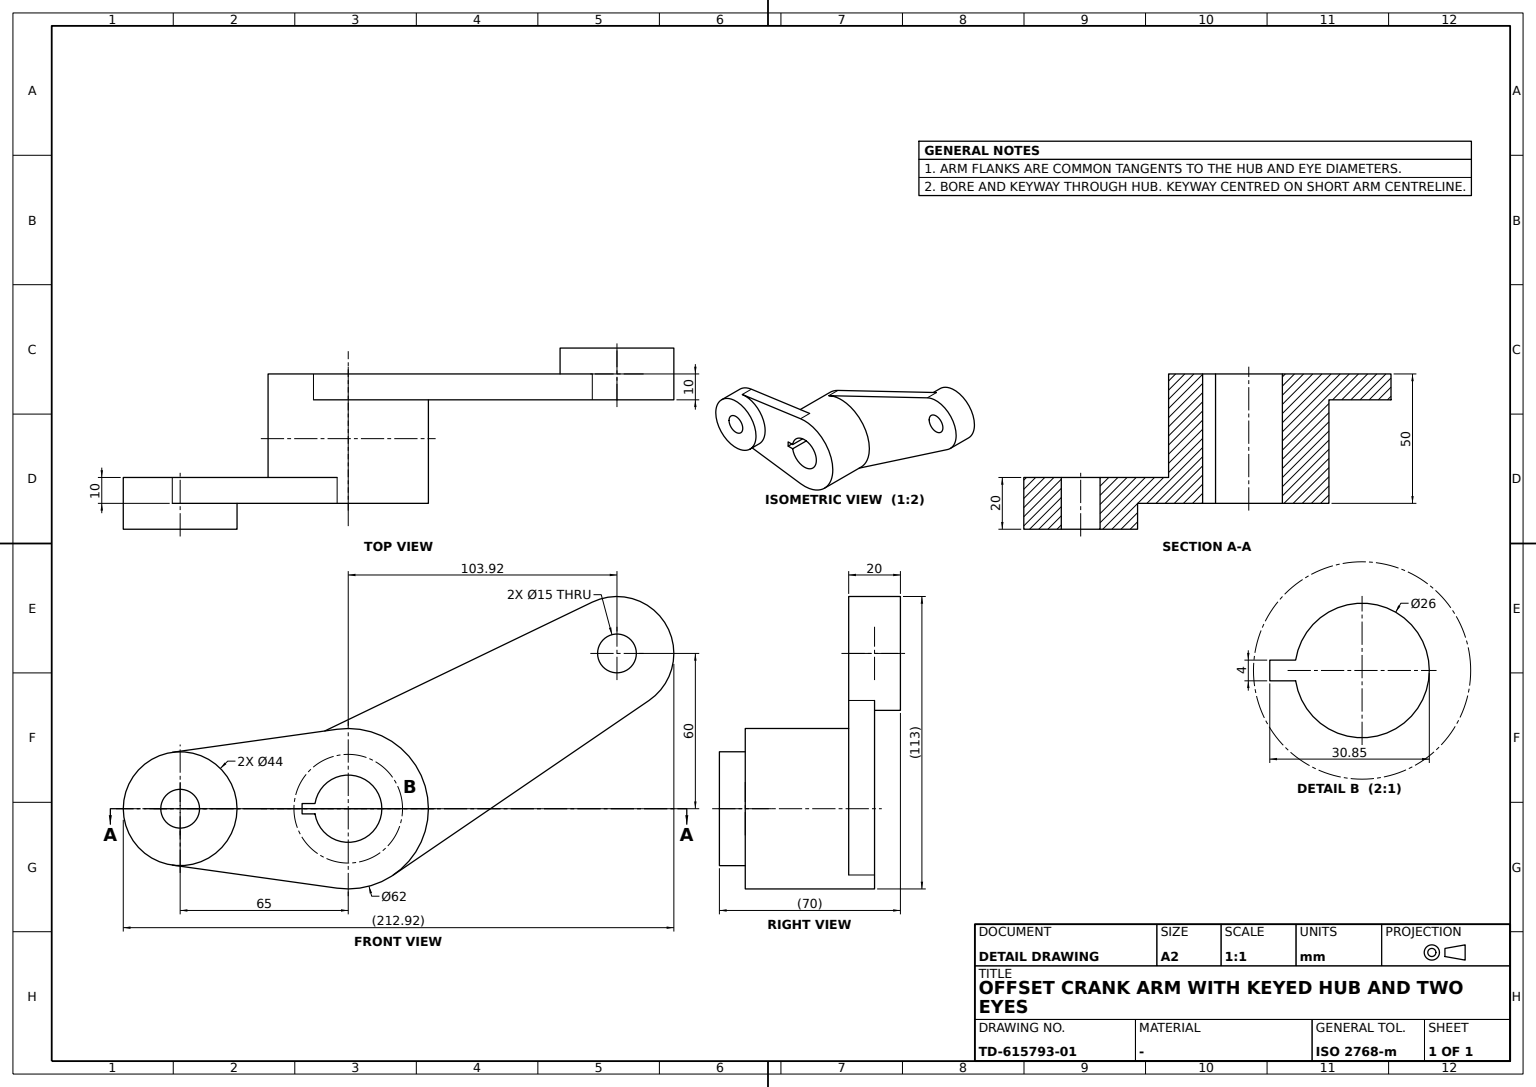
ISO-10303-21;
HEADER;
FILE_DESCRIPTION((''),'2;1');
FILE_NAME('','',(''),(''),'','','');
FILE_SCHEMA(('AUTOMOTIVE_DESIGN'));
ENDSEC;
DATA;
#1=APPLICATION_CONTEXT('');
#2=PRODUCT_CONTEXT('',#1,'mechanical');
#3=PRODUCT('','','',(#2));
#4=PRODUCT_DEFINITION_FORMATION('','',#3);
#5=PRODUCT_DEFINITION_CONTEXT('',#1,'design');
#6=PRODUCT_DEFINITION('','',#4,#5);
#7=PRODUCT_DEFINITION_SHAPE('','',#6);
#8=(LENGTH_UNIT()NAMED_UNIT(*)SI_UNIT(.MILLI.,.METRE.));
#9=(NAMED_UNIT(*)PLANE_ANGLE_UNIT()SI_UNIT($,.RADIAN.));
#10=(NAMED_UNIT(*)SI_UNIT($,.STERADIAN.)SOLID_ANGLE_UNIT());
#11=UNCERTAINTY_MEASURE_WITH_UNIT(LENGTH_MEASURE(0.005),#8,'distance_accuracy_value','');
#12=(GEOMETRIC_REPRESENTATION_CONTEXT(3)GLOBAL_UNCERTAINTY_ASSIGNED_CONTEXT((#11))GLOBAL_UNIT_ASSIGNED_CONTEXT((#8,#9,#10))REPRESENTATION_CONTEXT('',''));
#13=CARTESIAN_POINT('',(-17.469854,25.608674,10.));
#14=VERTEX_POINT('',#13);
#15=CARTESIAN_POINT('',(-17.469854,25.608674,0.));
#16=VERTEX_POINT('',#15);
#17=DIRECTION('',(0.,0.,-1.));
#18=VECTOR('',#17,1000.);
#19=LINE('',#13,#18);
#20=EDGE_CURVE('',#14,#16,#19,.T.);
#21=ORIENTED_EDGE('',*,*,#20,.T.);
#22=CARTESIAN_POINT('',(-116.321009,-41.826102,0.));
#23=VERTEX_POINT('',#22);
#24=DIRECTION('',(-0.826086272,-0.563543672,0.));
#25=VECTOR('',#24,1000.);
#26=LINE('',#15,#25);
#27=EDGE_CURVE('',#16,#23,#26,.T.);
#28=ORIENTED_EDGE('',*,*,#27,.T.);
#29=CARTESIAN_POINT('',(-116.321009,-41.826102,10.));
#30=VERTEX_POINT('',#29);
#31=LINE('',#29,#18);
#32=EDGE_CURVE('',#30,#23,#31,.T.);
#33=ORIENTED_EDGE('',*,*,#32,.F.);
#34=LINE('',#13,#25);
#35=EDGE_CURVE('',#14,#30,#34,.T.);
#36=ORIENTED_EDGE('',*,*,#35,.F.);
#37=EDGE_LOOP('',(#21,#28,#33,#36));
#38=FACE_BOUND('',#37,.T.);
#39=DIRECTION('',(0.563543672,-0.826086272,0.));
#40=DIRECTION('',(0.826086272,0.563543672,0.));
#41=AXIS2_PLACEMENT_3D('',#13,#39,#40);
#42=PLANE('',#41);
#43=ADVANCED_FACE('',(#38),#42,.F.);
#44=CARTESIAN_POINT('',(43.,0.,60.));
#45=VERTEX_POINT('',#44);
#46=CARTESIAN_POINT('',(87.,0.,60.));
#47=VERTEX_POINT('',#46);
#48=CARTESIAN_POINT('',(65.,0.,60.));
#49=DIRECTION('',(0.,0.,1.));
#50=DIRECTION('',(1.,0.,0.));
#51=AXIS2_PLACEMENT_3D('',#48,#49,#50);
#52=CIRCLE('',#51,22.);
#53=EDGE_CURVE('',#45,#47,#52,.T.);
#54=ORIENTED_EDGE('',*,*,#53,.F.);
#55=CARTESIAN_POINT('',(43.,0.,50.));
#56=VERTEX_POINT('',#55);
#57=CARTESIAN_POINT('',(43.,0.,40.));
#58=VECTOR('',#49,1000.);
#59=LINE('',#57,#58);
#60=EDGE_CURVE('',#45,#56,#59,.F.);
#61=ORIENTED_EDGE('',*,*,#60,.T.);
#62=CARTESIAN_POINT('',(68.046154,-21.788092,50.));
#63=VERTEX_POINT('',#62);
#64=CARTESIAN_POINT('',(65.,0.,50.));
#65=AXIS2_PLACEMENT_3D('',#64,#17,#50);
#66=CIRCLE('',#65,22.);
#67=EDGE_CURVE('',#63,#56,#66,.T.);
#68=ORIENTED_EDGE('',*,*,#67,.F.);
#69=CARTESIAN_POINT('',(68.046154,-21.788092,40.));
#70=VERTEX_POINT('',#69);
#71=LINE('',#69,#58);
#72=EDGE_CURVE('',#70,#63,#71,.T.);
#73=ORIENTED_EDGE('',*,*,#72,.F.);
#74=CARTESIAN_POINT('',(87.,0.,40.));
#75=VERTEX_POINT('',#74);
#76=CARTESIAN_POINT('',(65.,0.,40.));
#77=AXIS2_PLACEMENT_3D('',#76,#49,#50);
#78=CIRCLE('',#77,22.);
#79=EDGE_CURVE('',#70,#75,#78,.T.);
#80=ORIENTED_EDGE('',*,*,#79,.T.);
#81=LINE('',#74,#58);
#82=EDGE_CURVE('',#75,#47,#81,.T.);
#83=ORIENTED_EDGE('',*,*,#82,.T.);
#84=EDGE_LOOP('',(#54,#61,#68,#73,#80,#83));
#85=FACE_BOUND('',#84,.T.);
#86=CYLINDRICAL_SURFACE('',#77,22.);
#87=ADVANCED_FACE('',(#85),#86,.T.);
#88=CARTESIAN_POINT('',(68.046154,21.788092,40.));
#89=VERTEX_POINT('',#88);
#90=CARTESIAN_POINT('',(68.046154,21.788092,50.));
#91=VERTEX_POINT('',#90);
#92=LINE('',#88,#58);
#93=EDGE_CURVE('',#89,#91,#92,.T.);
#94=ORIENTED_EDGE('',*,*,#93,.T.);
#95=EDGE_CURVE('',#56,#91,#66,.T.);
#96=ORIENTED_EDGE('',*,*,#95,.F.);
#97=ORIENTED_EDGE('',*,*,#60,.F.);
#98=EDGE_CURVE('',#47,#45,#52,.T.);
#99=ORIENTED_EDGE('',*,*,#98,.F.);
#100=ORIENTED_EDGE('',*,*,#82,.F.);
#101=EDGE_CURVE('',#75,#89,#78,.T.);
#102=ORIENTED_EDGE('',*,*,#101,.T.);
#103=EDGE_LOOP('',(#94,#96,#97,#99,#100,#102));
#104=FACE_BOUND('',#103,.T.);
#105=ADVANCED_FACE('',(#104),#86,.T.);
#106=CARTESIAN_POINT('',(-94.382971,-79.823898,0.));
#107=VERTEX_POINT('',#106);
#108=CARTESIAN_POINT('',(13.442836,-27.933674,0.));
#109=VERTEX_POINT('',#108);
#110=DIRECTION('',(0.901086272,0.433639862,0.));
#111=VECTOR('',#110,1000.);
#112=LINE('',#106,#111);
#113=EDGE_CURVE('',#107,#109,#112,.T.);
#114=ORIENTED_EDGE('',*,*,#113,.F.);
#115=CARTESIAN_POINT('',(-81.923048,-60.,0.));
#116=VERTEX_POINT('',#115);
#117=CARTESIAN_POINT('',(-103.923048,-60.,0.));
#118=AXIS2_PLACEMENT_3D('',#117,#17,#50);
#119=CIRCLE('',#118,22.);
#120=EDGE_CURVE('',#116,#107,#119,.T.);
#121=ORIENTED_EDGE('',*,*,#120,.F.);
#122=EDGE_CURVE('',#23,#116,#119,.T.);
#123=ORIENTED_EDGE('',*,*,#122,.F.);
#124=ORIENTED_EDGE('',*,*,#27,.F.);
#125=CARTESIAN_POINT('',(31.,0.,0.));
#126=VERTEX_POINT('',#125);
#127=CARTESIAN_POINT('',(0.,0.,0.));
#128=AXIS2_PLACEMENT_3D('',#127,#49,#50);
#129=CIRCLE('',#128,31.);
#130=EDGE_CURVE('',#126,#16,#129,.T.);
#131=ORIENTED_EDGE('',*,*,#130,.F.);
#132=EDGE_CURVE('',#109,#126,#129,.T.);
#133=ORIENTED_EDGE('',*,*,#132,.F.);
#134=EDGE_LOOP('',(#114,#121,#123,#124,#131,#133));
#135=FACE_BOUND('',#134,.T.);
#136=CARTESIAN_POINT('',(17.845233,2.,0.));
#137=VERTEX_POINT('',#136);
#138=CARTESIAN_POINT('',(12.845233,2.,0.));
#139=VERTEX_POINT('',#138);
#140=DIRECTION('',(-1.,0.,0.));
#141=VECTOR('',#140,1000.);
#142=LINE('',#136,#141);
#143=EDGE_CURVE('',#137,#139,#142,.T.);
#144=ORIENTED_EDGE('',*,*,#143,.T.);
#145=CARTESIAN_POINT('',(12.845233,-2.,0.));
#146=VERTEX_POINT('',#145);
#147=CIRCLE('',#128,13.);
#148=EDGE_CURVE('',#139,#146,#147,.T.);
#149=ORIENTED_EDGE('',*,*,#148,.T.);
#150=CARTESIAN_POINT('',(17.845233,-2.,0.));
#151=VERTEX_POINT('',#150);
#152=VECTOR('',#50,1000.);
#153=LINE('',#145,#152);
#154=EDGE_CURVE('',#146,#151,#153,.T.);
#155=ORIENTED_EDGE('',*,*,#154,.T.);
#156=DIRECTION('',(0.,1.,0.));
#157=VECTOR('',#156,1000.);
#158=LINE('',#150,#157);
#159=EDGE_CURVE('',#151,#137,#158,.T.);
#160=ORIENTED_EDGE('',*,*,#159,.T.);
#161=EDGE_LOOP('',(#144,#149,#155,#160));
#162=FACE_BOUND('',#161,.T.);
#163=PLANE('',#128);
#164=ADVANCED_FACE('',(#135,#162),#163,.F.);
#165=CARTESIAN_POINT('',(-96.423048,-60.,10.));
#166=VERTEX_POINT('',#165);
#167=CARTESIAN_POINT('',(-111.423048,-60.,10.));
#168=VERTEX_POINT('',#167);
#169=CARTESIAN_POINT('',(-103.923048,-60.,10.));
#170=AXIS2_PLACEMENT_3D('',#169,#17,#140);
#171=CIRCLE('',#170,7.5);
#172=EDGE_CURVE('',#166,#168,#171,.T.);
#173=ORIENTED_EDGE('',*,*,#172,.F.);
#174=CARTESIAN_POINT('',(-96.423048,-60.,-10.));
#175=VERTEX_POINT('',#174);
#176=LINE('',#165,#18);
#177=EDGE_CURVE('',#166,#175,#176,.T.);
#178=ORIENTED_EDGE('',*,*,#177,.T.);
#179=CARTESIAN_POINT('',(-111.423048,-60.,-10.));
#180=VERTEX_POINT('',#179);
#181=CARTESIAN_POINT('',(-103.923048,-60.,-10.));
#182=AXIS2_PLACEMENT_3D('',#181,#17,#140);
#183=CIRCLE('',#182,7.5);
#184=EDGE_CURVE('',#175,#180,#183,.T.);
#185=ORIENTED_EDGE('',*,*,#184,.T.);
#186=LINE('',#167,#18);
#187=EDGE_CURVE('',#180,#168,#186,.F.);
#188=ORIENTED_EDGE('',*,*,#187,.T.);
#189=EDGE_LOOP('',(#173,#178,#185,#188));
#190=FACE_BOUND('',#189,.T.);
#191=CYLINDRICAL_SURFACE('',#170,7.5);
#192=ADVANCED_FACE('',(#190),#191,.F.);
#193=CARTESIAN_POINT('',(-94.382971,-79.823898,10.));
#194=VERTEX_POINT('',#193);
#195=LINE('',#193,#18);
#196=EDGE_CURVE('',#194,#107,#195,.T.);
#197=ORIENTED_EDGE('',*,*,#196,.F.);
#198=CARTESIAN_POINT('',(-125.923048,-60.,10.));
#199=VERTEX_POINT('',#198);
#200=AXIS2_PLACEMENT_3D('',#169,#49,#50);
#201=CIRCLE('',#200,22.);
#202=EDGE_CURVE('',#199,#194,#201,.T.);
#203=ORIENTED_EDGE('',*,*,#202,.F.);
#204=CARTESIAN_POINT('',(-125.923048,-60.,-10.));
#205=VERTEX_POINT('',#204);
#206=LINE('',#198,#18);
#207=EDGE_CURVE('',#205,#199,#206,.F.);
#208=ORIENTED_EDGE('',*,*,#207,.F.);
#209=CARTESIAN_POINT('',(-81.923048,-60.,-10.));
#210=VERTEX_POINT('',#209);
#211=AXIS2_PLACEMENT_3D('',#181,#49,#50);
#212=CIRCLE('',#211,22.);
#213=EDGE_CURVE('',#205,#210,#212,.T.);
#214=ORIENTED_EDGE('',*,*,#213,.T.);
#215=CARTESIAN_POINT('',(-81.923048,-60.,10.));
#216=LINE('',#215,#18);
#217=EDGE_CURVE('',#116,#210,#216,.T.);
#218=ORIENTED_EDGE('',*,*,#217,.F.);
#219=ORIENTED_EDGE('',*,*,#120,.T.);
#220=EDGE_LOOP('',(#197,#203,#208,#214,#218,#219));
#221=FACE_BOUND('',#220,.T.);
#222=CYLINDRICAL_SURFACE('',#170,22.);
#223=ADVANCED_FACE('',(#221),#222,.T.);
#224=CARTESIAN_POINT('',(72.5,0.,40.));
#225=VERTEX_POINT('',#224);
#226=CARTESIAN_POINT('',(57.5,0.,40.));
#227=VERTEX_POINT('',#226);
#228=AXIS2_PLACEMENT_3D('',#76,#17,#140);
#229=CIRCLE('',#228,7.5);
#230=EDGE_CURVE('',#225,#227,#229,.T.);
#231=ORIENTED_EDGE('',*,*,#230,.F.);
#232=EDGE_CURVE('',#227,#225,#229,.T.);
#233=ORIENTED_EDGE('',*,*,#232,.F.);
#234=EDGE_LOOP('',(#231,#233));
#235=FACE_BOUND('',#234,.T.);
#236=CARTESIAN_POINT('',(4.292308,30.701402,40.));
#237=VERTEX_POINT('',#236);
#238=DIRECTION('',(-0.990367812,0.138461538,0.));
#239=VECTOR('',#238,1000.);
#240=LINE('',#88,#239);
#241=EDGE_CURVE('',#89,#237,#240,.T.);
#242=ORIENTED_EDGE('',*,*,#241,.F.);
#243=ORIENTED_EDGE('',*,*,#101,.F.);
#244=ORIENTED_EDGE('',*,*,#79,.F.);
#245=CARTESIAN_POINT('',(4.292308,-30.701402,40.));
#246=VERTEX_POINT('',#245);
#247=DIRECTION('',(0.990367812,0.138461538,0.));
#248=VECTOR('',#247,1000.);
#249=LINE('',#245,#248);
#250=EDGE_CURVE('',#246,#70,#249,.T.);
#251=ORIENTED_EDGE('',*,*,#250,.F.);
#252=CARTESIAN_POINT('',(31.,0.,40.));
#253=VERTEX_POINT('',#252);
#254=CARTESIAN_POINT('',(0.,0.,40.));
#255=AXIS2_PLACEMENT_3D('',#254,#17,#50);
#256=CIRCLE('',#255,31.);
#257=EDGE_CURVE('',#253,#246,#256,.T.);
#258=ORIENTED_EDGE('',*,*,#257,.F.);
#259=EDGE_CURVE('',#237,#253,#256,.T.);
#260=ORIENTED_EDGE('',*,*,#259,.F.);
#261=EDGE_LOOP('',(#242,#243,#244,#251,#258,#260));
#262=FACE_BOUND('',#261,.T.);
#263=AXIS2_PLACEMENT_3D('',#254,#17,#140);
#264=PLANE('',#263);
#265=ADVANCED_FACE('',(#235,#262),#264,.T.);
#266=ORIENTED_EDGE('',*,*,#196,.T.);
#267=ORIENTED_EDGE('',*,*,#113,.T.);
#268=CARTESIAN_POINT('',(13.442836,-27.933674,10.));
#269=VERTEX_POINT('',#268);
#270=LINE('',#268,#18);
#271=EDGE_CURVE('',#269,#109,#270,.T.);
#272=ORIENTED_EDGE('',*,*,#271,.F.);
#273=LINE('',#193,#111);
#274=EDGE_CURVE('',#194,#269,#273,.T.);
#275=ORIENTED_EDGE('',*,*,#274,.F.);
#276=EDGE_LOOP('',(#266,#267,#272,#275));
#277=FACE_BOUND('',#276,.T.);
#278=DIRECTION('',(-0.433639862,0.901086272,0.));
#279=DIRECTION('',(-0.901086272,-0.433639862,0.));
#280=AXIS2_PLACEMENT_3D('',#193,#278,#279);
#281=PLANE('',#280);
#282=ADVANCED_FACE('',(#277),#281,.F.);
#283=CARTESIAN_POINT('',(17.845233,2.,50.));
#284=VERTEX_POINT('',#283);
#285=LINE('',#136,#18);
#286=EDGE_CURVE('',#284,#137,#285,.T.);
#287=ORIENTED_EDGE('',*,*,#286,.T.);
#288=ORIENTED_EDGE('',*,*,#159,.F.);
#289=CARTESIAN_POINT('',(17.845233,-2.,50.));
#290=VERTEX_POINT('',#289);
#291=LINE('',#150,#18);
#292=EDGE_CURVE('',#290,#151,#291,.T.);
#293=ORIENTED_EDGE('',*,*,#292,.F.);
#294=LINE('',#289,#157);
#295=EDGE_CURVE('',#290,#284,#294,.T.);
#296=ORIENTED_EDGE('',*,*,#295,.T.);
#297=EDGE_LOOP('',(#287,#288,#293,#296));
#298=FACE_BOUND('',#297,.T.);
#299=AXIS2_PLACEMENT_3D('',#150,#50,#17);
#300=PLANE('',#299);
#301=ADVANCED_FACE('',(#298),#300,.F.);
#302=EDGE_CURVE('',#180,#175,#183,.T.);
#303=ORIENTED_EDGE('',*,*,#302,.F.);
#304=ORIENTED_EDGE('',*,*,#184,.F.);
#305=EDGE_LOOP('',(#303,#304));
#306=FACE_BOUND('',#305,.T.);
#307=ORIENTED_EDGE('',*,*,#213,.F.);
#308=EDGE_CURVE('',#210,#205,#212,.T.);
#309=ORIENTED_EDGE('',*,*,#308,.F.);
#310=EDGE_LOOP('',(#307,#309));
#311=FACE_BOUND('',#310,.T.);
#312=PLANE('',#182);
#313=ADVANCED_FACE('',(#306,#311),#312,.T.);
#314=ORIENTED_EDGE('',*,*,#217,.T.);
#315=ORIENTED_EDGE('',*,*,#308,.T.);
#316=ORIENTED_EDGE('',*,*,#207,.T.);
#317=EDGE_CURVE('',#30,#199,#201,.T.);
#318=ORIENTED_EDGE('',*,*,#317,.F.);
#319=ORIENTED_EDGE('',*,*,#32,.T.);
#320=ORIENTED_EDGE('',*,*,#122,.T.);
#321=EDGE_LOOP('',(#314,#315,#316,#318,#319,#320));
#322=FACE_BOUND('',#321,.T.);
#323=ADVANCED_FACE('',(#322),#222,.T.);
#324=ORIENTED_EDGE('',*,*,#130,.T.);
#325=ORIENTED_EDGE('',*,*,#20,.F.);
#326=CARTESIAN_POINT('',(-31.,0.,10.));
#327=VERTEX_POINT('',#326);
#328=CARTESIAN_POINT('',(0.,0.,10.));
#329=AXIS2_PLACEMENT_3D('',#328,#17,#50);
#330=CIRCLE('',#329,31.);
#331=EDGE_CURVE('',#327,#14,#330,.T.);
#332=ORIENTED_EDGE('',*,*,#331,.F.);
#333=CARTESIAN_POINT('',(-31.,0.,50.));
#334=VERTEX_POINT('',#333);
#335=LINE('',#333,#18);
#336=EDGE_CURVE('',#327,#334,#335,.F.);
#337=ORIENTED_EDGE('',*,*,#336,.T.);
#338=CARTESIAN_POINT('',(4.292308,30.701402,50.));
#339=VERTEX_POINT('',#338);
#340=CARTESIAN_POINT('',(0.,0.,50.));
#341=AXIS2_PLACEMENT_3D('',#340,#49,#50);
#342=CIRCLE('',#341,31.);
#343=EDGE_CURVE('',#339,#334,#342,.T.);
#344=ORIENTED_EDGE('',*,*,#343,.F.);
#345=LINE('',#236,#58);
#346=EDGE_CURVE('',#237,#339,#345,.T.);
#347=ORIENTED_EDGE('',*,*,#346,.F.);
#348=ORIENTED_EDGE('',*,*,#259,.T.);
#349=CARTESIAN_POINT('',(31.,0.,50.));
#350=LINE('',#349,#18);
#351=EDGE_CURVE('',#253,#126,#350,.T.);
#352=ORIENTED_EDGE('',*,*,#351,.T.);
#353=EDGE_LOOP('',(#324,#325,#332,#337,#344,#347,#348,#352));
#354=FACE_BOUND('',#353,.T.);
#355=AXIS2_PLACEMENT_3D('',#340,#17,#140);
#356=CYLINDRICAL_SURFACE('',#355,31.);
#357=ADVANCED_FACE('',(#354),#356,.T.);
#358=ORIENTED_EDGE('',*,*,#53,.T.);
#359=ORIENTED_EDGE('',*,*,#98,.T.);
#360=EDGE_LOOP('',(#358,#359));
#361=FACE_BOUND('',#360,.T.);
#362=CARTESIAN_POINT('',(72.5,0.,60.));
#363=VERTEX_POINT('',#362);
#364=CARTESIAN_POINT('',(57.5,0.,60.));
#365=VERTEX_POINT('',#364);
#366=AXIS2_PLACEMENT_3D('',#48,#17,#140);
#367=CIRCLE('',#366,7.5);
#368=EDGE_CURVE('',#363,#365,#367,.T.);
#369=ORIENTED_EDGE('',*,*,#368,.T.);
#370=EDGE_CURVE('',#365,#363,#367,.T.);
#371=ORIENTED_EDGE('',*,*,#370,.T.);
#372=EDGE_LOOP('',(#369,#371));
#373=FACE_BOUND('',#372,.T.);
#374=PLANE('',#51);
#375=ADVANCED_FACE('',(#361,#373),#374,.T.);
#376=LINE('',#362,#18);
#377=EDGE_CURVE('',#363,#225,#376,.T.);
#378=ORIENTED_EDGE('',*,*,#377,.T.);
#379=ORIENTED_EDGE('',*,*,#230,.T.);
#380=LINE('',#364,#18);
#381=EDGE_CURVE('',#227,#365,#380,.F.);
#382=ORIENTED_EDGE('',*,*,#381,.T.);
#383=ORIENTED_EDGE('',*,*,#368,.F.);
#384=EDGE_LOOP('',(#378,#379,#382,#383));
#385=FACE_BOUND('',#384,.T.);
#386=CYLINDRICAL_SURFACE('',#366,7.5);
#387=ADVANCED_FACE('',(#385),#386,.F.);
#388=ORIENTED_EDGE('',*,*,#292,.T.);
#389=ORIENTED_EDGE('',*,*,#154,.F.);
#390=CARTESIAN_POINT('',(12.845233,-2.,50.));
#391=VERTEX_POINT('',#390);
#392=LINE('',#145,#18);
#393=EDGE_CURVE('',#391,#146,#392,.T.);
#394=ORIENTED_EDGE('',*,*,#393,.F.);
#395=LINE('',#390,#152);
#396=EDGE_CURVE('',#391,#290,#395,.T.);
#397=ORIENTED_EDGE('',*,*,#396,.T.);
#398=EDGE_LOOP('',(#388,#389,#394,#397));
#399=FACE_BOUND('',#398,.T.);
#400=DIRECTION('',(0.,-1.,0.));
#401=AXIS2_PLACEMENT_3D('',#145,#400,#17);
#402=PLANE('',#401);
#403=ADVANCED_FACE('',(#399),#402,.F.);
#404=CARTESIAN_POINT('',(4.292308,-30.701402,50.));
#405=VERTEX_POINT('',#404);
#406=EDGE_CURVE('',#334,#405,#342,.T.);
#407=ORIENTED_EDGE('',*,*,#406,.F.);
#408=ORIENTED_EDGE('',*,*,#336,.F.);
#409=EDGE_CURVE('',#269,#327,#330,.T.);
#410=ORIENTED_EDGE('',*,*,#409,.F.);
#411=ORIENTED_EDGE('',*,*,#271,.T.);
#412=ORIENTED_EDGE('',*,*,#132,.T.);
#413=ORIENTED_EDGE('',*,*,#351,.F.);
#414=ORIENTED_EDGE('',*,*,#257,.T.);
#415=LINE('',#245,#58);
#416=EDGE_CURVE('',#246,#405,#415,.T.);
#417=ORIENTED_EDGE('',*,*,#416,.T.);
#418=EDGE_LOOP('',(#407,#408,#410,#411,#412,#413,#414,#417));
#419=FACE_BOUND('',#418,.T.);
#420=ADVANCED_FACE('',(#419),#356,.T.);
#421=ORIENTED_EDGE('',*,*,#67,.T.);
#422=ORIENTED_EDGE('',*,*,#95,.T.);
#423=LINE('',#90,#239);
#424=EDGE_CURVE('',#91,#339,#423,.T.);
#425=ORIENTED_EDGE('',*,*,#424,.T.);
#426=ORIENTED_EDGE('',*,*,#343,.T.);
#427=ORIENTED_EDGE('',*,*,#406,.T.);
#428=LINE('',#404,#248);
#429=EDGE_CURVE('',#405,#63,#428,.T.);
#430=ORIENTED_EDGE('',*,*,#429,.T.);
#431=EDGE_LOOP('',(#421,#422,#425,#426,#427,#430));
#432=FACE_BOUND('',#431,.T.);
#433=ORIENTED_EDGE('',*,*,#396,.F.);
#434=CARTESIAN_POINT('',(12.845233,2.,50.));
#435=VERTEX_POINT('',#434);
#436=CIRCLE('',#341,13.);
#437=EDGE_CURVE('',#435,#391,#436,.T.);
#438=ORIENTED_EDGE('',*,*,#437,.F.);
#439=LINE('',#283,#141);
#440=EDGE_CURVE('',#284,#435,#439,.T.);
#441=ORIENTED_EDGE('',*,*,#440,.F.);
#442=ORIENTED_EDGE('',*,*,#295,.F.);
#443=EDGE_LOOP('',(#433,#438,#441,#442));
#444=FACE_BOUND('',#443,.T.);
#445=PLANE('',#341);
#446=ADVANCED_FACE('',(#432,#444),#445,.T.);
#447=ORIENTED_EDGE('',*,*,#241,.T.);
#448=ORIENTED_EDGE('',*,*,#346,.T.);
#449=ORIENTED_EDGE('',*,*,#424,.F.);
#450=ORIENTED_EDGE('',*,*,#93,.F.);
#451=EDGE_LOOP('',(#447,#448,#449,#450));
#452=FACE_BOUND('',#451,.T.);
#453=DIRECTION('',(0.138461538,0.990367812,0.));
#454=AXIS2_PLACEMENT_3D('',#88,#453,#238);
#455=PLANE('',#454);
#456=ADVANCED_FACE('',(#452),#455,.T.);
#457=ORIENTED_EDGE('',*,*,#72,.T.);
#458=ORIENTED_EDGE('',*,*,#429,.F.);
#459=ORIENTED_EDGE('',*,*,#416,.F.);
#460=ORIENTED_EDGE('',*,*,#250,.T.);
#461=EDGE_LOOP('',(#457,#458,#459,#460));
#462=FACE_BOUND('',#461,.T.);
#463=DIRECTION('',(0.138461538,-0.990367812,0.));
#464=AXIS2_PLACEMENT_3D('',#245,#463,#247);
#465=PLANE('',#464);
#466=ADVANCED_FACE('',(#462),#465,.T.);
#467=LINE('',#138,#18);
#468=EDGE_CURVE('',#435,#139,#467,.T.);
#469=ORIENTED_EDGE('',*,*,#468,.T.);
#470=ORIENTED_EDGE('',*,*,#143,.F.);
#471=ORIENTED_EDGE('',*,*,#286,.F.);
#472=ORIENTED_EDGE('',*,*,#440,.T.);
#473=EDGE_LOOP('',(#469,#470,#471,#472));
#474=FACE_BOUND('',#473,.T.);
#475=AXIS2_PLACEMENT_3D('',#136,#156,#49);
#476=PLANE('',#475);
#477=ADVANCED_FACE('',(#474),#476,.F.);
#478=ORIENTED_EDGE('',*,*,#437,.T.);
#479=ORIENTED_EDGE('',*,*,#393,.T.);
#480=ORIENTED_EDGE('',*,*,#148,.F.);
#481=ORIENTED_EDGE('',*,*,#468,.F.);
#482=EDGE_LOOP('',(#478,#479,#480,#481));
#483=FACE_BOUND('',#482,.T.);
#484=CYLINDRICAL_SURFACE('',#128,13.);
#485=ADVANCED_FACE('',(#483),#484,.F.);
#486=ORIENTED_EDGE('',*,*,#187,.F.);
#487=ORIENTED_EDGE('',*,*,#302,.T.);
#488=ORIENTED_EDGE('',*,*,#177,.F.);
#489=EDGE_CURVE('',#168,#166,#171,.T.);
#490=ORIENTED_EDGE('',*,*,#489,.F.);
#491=EDGE_LOOP('',(#486,#487,#488,#490));
#492=FACE_BOUND('',#491,.T.);
#493=ADVANCED_FACE('',(#492),#191,.F.);
#494=ORIENTED_EDGE('',*,*,#232,.T.);
#495=ORIENTED_EDGE('',*,*,#377,.F.);
#496=ORIENTED_EDGE('',*,*,#370,.F.);
#497=ORIENTED_EDGE('',*,*,#381,.F.);
#498=EDGE_LOOP('',(#494,#495,#496,#497));
#499=FACE_BOUND('',#498,.T.);
#500=ADVANCED_FACE('',(#499),#386,.F.);
#501=ORIENTED_EDGE('',*,*,#489,.T.);
#502=ORIENTED_EDGE('',*,*,#172,.T.);
#503=EDGE_LOOP('',(#501,#502));
#504=FACE_BOUND('',#503,.T.);
#505=ORIENTED_EDGE('',*,*,#409,.T.);
#506=ORIENTED_EDGE('',*,*,#331,.T.);
#507=ORIENTED_EDGE('',*,*,#35,.T.);
#508=ORIENTED_EDGE('',*,*,#317,.T.);
#509=ORIENTED_EDGE('',*,*,#202,.T.);
#510=ORIENTED_EDGE('',*,*,#274,.T.);
#511=EDGE_LOOP('',(#505,#506,#507,#508,#509,#510));
#512=FACE_BOUND('',#511,.T.);
#513=PLANE('',#200);
#514=ADVANCED_FACE('',(#504,#512),#513,.T.);
#515=CLOSED_SHELL('',(#43,#87,#105,#164,#192,#223,#265,#282,#301,#313,#323,#357,#375,#387,#403,#420,#446,#456,#466,#477,#485,#493,#500,#514));
#516=MANIFOLD_SOLID_BREP('',#515);
#517=ADVANCED_BREP_SHAPE_REPRESENTATION('',(#516),#12);
#518=SHAPE_DEFINITION_REPRESENTATION(#7,#517);
ENDSEC;
END-ISO-10303-21;
